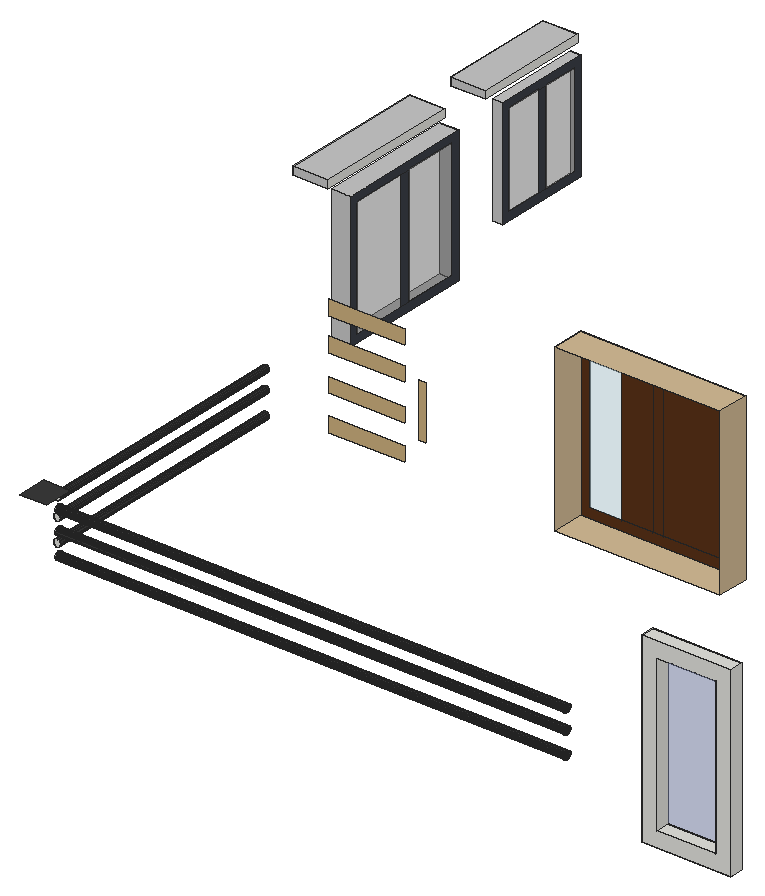
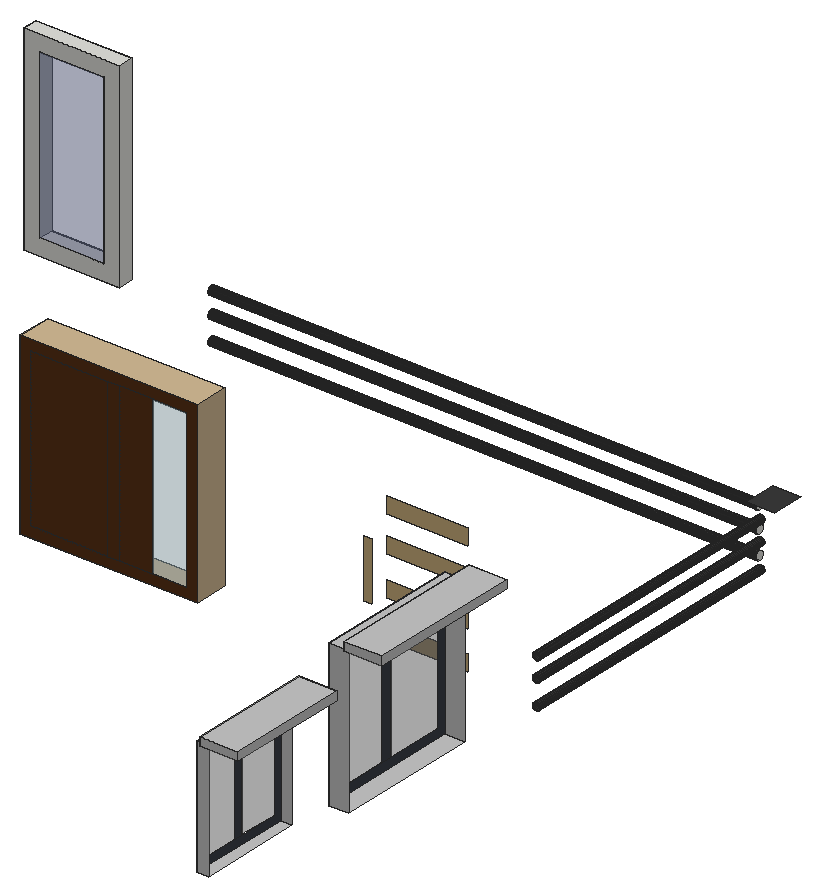
# SketchUp Ruby script. Lengths in inches.
U = 1.inch
M = Sketchup.active_model
def pt(a) = Geom::Point3d.new(a.map { |v| v * U })
def face(e, loops, mat)
  f = e.add_face(loops[0].map { |a| pt(a) })
  loops[1..].each { |l| e.add_face(l.map { |a| pt(a) }).erase! }
  f.material = f.back_material = mat if mat
  f
end
# faces: each face lists its corners as indices into pts; further lists are holes
def faces(e, pts, list, mat = nil) = list.each { |f| face(e, (f[0].is_a?(Array) ? f : [f]).map { |l| l.map { |i| pts[i] } }, mat) }
# xy, xz, yz: faces in a plane at the given z, y or x. An outline is a flat list of corners, or four numbers for a rectangle; further outlines are holes
def ring(l) = l.size == 4 ? [[l[0], l[1]], [l[2], l[1]], [l[2], l[3]], [l[0], l[3]]] : l.each_slice(2).to_a
def flat(e, list, mat, &to3) = list.each { |f| face(e, (f[0].is_a?(Array) ? f : [f]).map { |l| ring(l).map { |u, v| to3.(u, v) } }, mat) }
def xy(e, z, list, mat = nil) = flat(e, list, mat) { |x, y| [x, y, z] }
def xz(e, y, list, mat = nil) = flat(e, list, mat) { |x, z| [x, y, z] }
def yz(e, x, list, mat = nil) = flat(e, list, mat) { |y, z| [x, y, z] }
def lines(e, pts, list) = list.each { |a, b| e.add_line(pt(pts[a]), pt(pts[b])) }
# prism: a flat outline (further loops are holes) pulled along v
def prism(e, loops, v, mat = nil)
  f = face(e, loops, mat); d = Geom::Vector3d.new(v.map { |x| x * U })
  f.pushpull(f.normal.samedirection?(d) ? d.length : -d.length)
end
def box(e, o, s, mat = nil) = prism(e, [[o, [o[0] + s[0], o[1], o[2]], [o[0] + s[0], o[1] + s[1], o[2]], [o[0], o[1] + s[1], o[2]]]], [0, 0, s[2]], mat)
def at(x, y, z, deg = 0) = Geom::Transformation.translation(pt([x, y, z])) * Geom::Transformation.rotation(ORIGIN, Z_AXIS, deg.degrees)
def axes(o, x, y, z) = Geom::Transformation.new([*x, 0, *y, 0, *z, 0, *pt(o).to_a, 1])
def part(name) = M.definitions.add(name)
# library, detail: a bought-in or finely detailed component or shape, given as its bounding box
def library(name, o, s) = part(name).tap { |d| box(d.entities, o, s) }
def detail(e, o, s) = box(e.add_group.entities, o, s)
def put(e, d, t, mat = nil) = e.add_instance(d, t).tap { |i| i.material = mat if mat }
def group(e, t, mat = nil) = e.add_group.tap { |g| g.transformation = t; g.material = mat if mat }.entities
root = M.entities
M.materials.add("[Color M02]").color = [198, 198, 198]
M.materials.add("[Color M07]").color = [58, 58, 58]
M.materials.add("[Formica Beige]").color = [211, 187, 149]
M.materials.add("[Formica Laminate Dark]").color = [59, 63, 71]
M.materials.add("[Translucent Glass Gray]").color = [128, 128, 128]
M.materials["[Translucent Glass Gray]"].alpha = 0.5
M.materials.add("[Translucent Glass Safety]").color = [204, 235, 244]
M.materials["[Translucent Glass Safety]"].alpha = 0.5
M.materials.add("[Translucent Glass Sky Reflection]").color = [126, 138, 183]
M.materials["[Translucent Glass Sky Reflection]"].alpha = 0.52
M.materials.add("[Wood Cherry Original]").color = [89, 50, 24]
M.materials.add("[Wood Floor Light]").color = [204, 176, 127]
xy(root,406.1,[[374.52,386.84,415.58,393.34]])
xy(root,411.53,[[213.51,538.2,289.58,552.88]],"[Formica Beige]")
xy(root,412.93,[[381.35,386.84,408.75,393.34]])
xy(root,421.07,[[73.92,584.23,82.36,646.54]],"[Color M02]")
xy(root,429.73,[[73.92,676.68,78.67,721.56]],"[Color M02]")
xy(root,431,[[79.95,477.84,80.34,477.9,80.7,478.05,81.01,478.28,81.25,478.59,81.4,478.96,81.45,479.34,81.4,479.73,81.25,480.09,81.01,480.41,80.7,480.64,80.34,480.79,79.95,480.84,79.5625,480.79,79.2,480.64,78.89,480.41,78.65,480.09,78.5,479.73,78.45,479.34,78.5,478.96,78.65,478.59,78.89,478.28,79.2,478.05,79.5625,477.9]])
xy(root,431.16,[[79.95,444.41,80.34,444.46,80.7,444.61,81.01,444.85,81.25,445.16,81.4,445.52,81.45,445.91,81.4,446.3,81.25,446.66,81.01,446.97,80.7,447.21,80.34,447.36,79.95,447.41,79.5625,447.36,79.2,447.21,78.89,446.97,78.65,446.66,78.5,446.3,78.45,445.91,78.5,445.52,78.65,445.16,78.89,444.85,79.2,444.61,79.5625,444.46]])
xy(root,431.4375,[[193.34,408.87,193.78,408.93,194.18,409.1,194.53,409.36,194.8,409.71,194.97,410.12,195.03,410.56,194.97,410.99,194.8,411.4,194.53,411.75,194.18,412.02,193.78,412.1875,193.34,412.25,192.9,412.1875,192.5,412.02,192.15,411.75,191.88,411.4,191.71,410.99,191.65,410.56,191.71,410.12,191.88,409.71,192.15,409.36,192.5,409.1,192.9,408.93]])
xy(root,431.5625,[[259.47,408.87,259.9,408.93,260.31,409.1,260.66,409.36,260.93,409.71,261.1,410.12,261.15,410.56,261.1,410.99,260.93,411.4,260.66,411.75,260.31,412.02,259.9,412.1875,259.47,412.25,259.03,412.1875,258.62,412.02,258.27,411.75,258,411.4,257.84,410.99,257.78,410.56,257.84,410.12,258,409.71,258.27,409.36,258.62,409.1,259.03,408.93]])
xy(root,431.75,[[128.47,408.87,128.9,408.93,129.31,409.1,129.66,409.36,129.93,409.71,130.1,410.12,130.15,410.56,130.1,410.99,129.93,411.4,129.66,411.75,129.31,412.02,128.9,412.1875,128.47,412.25,128.03,412.1875,127.62,412.02,127.27,411.75,127,411.4,126.84,410.99,126.78,410.56,126.84,410.12,127,409.71,127.27,409.36,127.62,409.1,128.03,408.93]])
xy(root,431.875,[[79.95,511.66,80.34,511.71,80.7,511.86,81.01,512.1,81.25,512.41,81.4,512.77,81.45,513.16,81.4,513.55,81.25,513.91,81.01,514.22,80.7,514.46,80.34,514.61,79.95,514.66,79.5625,514.61,79.2,514.46,78.89,514.22,78.65,513.91,78.5,513.55,78.45,513.16,78.5,512.77,78.65,512.41,78.89,512.1,79.2,511.86,79.5625,511.71]])
xy(root,436.0625,[[73.92,404.34,85.98,418.04]],"[Color M07]")
xy(root,480.23,[[73.92,676.68,78.67,721.56]],"[Color M02]")
xy(root,481.56,[[57.67,672.99,73.92,725.89]],"[Color M02]")
xy(root,483.38,[[73.92,584.23,82.36,646.54]],"[Color M02]")
xy(root,484.43,[[57.67,581.95,73.92,649.2]],"[Color M02]")
xy(root,484.52,[[381.35,386.84,408.75,393.34]])
xy(root,485.25,[[57.67,672.99,73.92,725.89]],"[Color M02]")
xy(root,487.59,[[213.51,538.2,289.58,552.88]],"[Formica Beige]")
xy(root,488.12,[[57.67,581.95,73.92,649.2]],"[Color M02]")
xy(root,491.35,[[374.52,386.84,415.58,393.34]])
xz(root,386.84,[[[374.52,406.1,415.58,491.35],[381.35,412.93,408.75,484.52]]])
xz(root,393.34,[[[374.52,406.1,415.58,491.35],[381.35,412.93,408.75,484.52]]])
xz(root,393.34,[[381.35,412.93,408.75,484.52]],"[Translucent Glass Sky Reflection]")
xz(root,418.04,[[80,410.64,80.42,410.7,80.81,410.86,81.15,411.12,81.4,411.45,81.57,411.85,81.62,412.27,81.57,412.6875,81.4,413.08,81.15,413.42,80.81,413.67,80.42,413.84,80,413.89,79.58,413.84,79.18,413.67,78.85,413.42,78.59,413.08,78.43,412.6875,78.37,412.27,78.43,411.85,78.59,411.45,78.85,411.12,79.18,410.86,79.58,410.7],[80,421.33,80.42,421.39,80.81,421.55,81.15,421.81,81.4,422.14,81.57,422.53,81.62,422.95,81.57,423.375,81.4,423.77,81.15,424.1,80.81,424.36,80.42,424.52,80,424.58,79.58,424.52,79.18,424.36,78.85,424.1,78.59,423.77,78.43,423.375,78.37,422.95,78.43,422.53,78.59,422.14,78.85,421.81,79.18,421.55,79.58,421.39],[80,429.95,80.42,430.01,80.81,430.17,81.15,430.43,81.4,430.77,81.57,431.16,81.62,431.58,81.57,432,81.4,432.39,81.15,432.73,80.81,432.99,80.42,433.15,80,433.2,79.58,433.15,79.18,432.99,78.85,432.73,78.59,432.39,78.43,432,78.37,431.58,78.43,431.16,78.59,430.77,78.85,430.43,79.18,430.17,79.58,430.01]])
xz(root,538.2,[[109.29,415.48,144.04,422.29],[150.7,427.01,154.02,451.83],[109.29,431.66,144.04,438.48],[109.29,448.48,144.04,455.29],[109.29,463.85,144.04,470.66]],"[Wood Floor Light]")
xz(root,552.88,[[217.97,415.98,232.47,483.13]],"[Translucent Glass Safety]")
xz(root,552.88,[[[213.51,411.53,289.58,487.59],[217.97,415.98,285.12,483.13]],[232.47,415.98,246.96,483.13],[246.96,415.98,251.87,483.13],[251.87,415.98,285.12,483.13]],"[Wood Cherry Original]")
xz(root,581.95,[[57.67,484.43,73.92,488.12]],"[Color M02]")
xz(root,584.23,[[73.92,421.07,82.36,483.38]],"[Color M02]")
xz(root,646.54,[[73.92,421.07,82.36,483.38]],"[Color M02]")
xz(root,649.2,[[57.67,484.43,73.92,488.12]],"[Color M02]")
xz(root,672.99,[[57.67,481.56,73.92,485.25]],"[Color M02]")
xz(root,676.68,[[73.92,429.73,78.67,480.23]],"[Color M02]")
xz(root,721.56,[[73.92,429.73,78.67,480.23]],"[Color M02]")
xz(root,725.89,[[57.67,481.56,73.92,485.25]],"[Color M02]")
yz(root,57.67,[[672.99,481.56,725.89,485.25],[581.95,484.43,649.2,488.12]],"[Color M02]")
yz(root,73.92,[[672.99,481.56,725.89,485.25],[581.95,484.43,649.2,488.12]])
yz(root,78.67,[[[676.68,429.73,721.56,480.23],[680.29,433.34,717.95,476.63]],[697.6,433.34,701.4,476.63]],"[Formica Laminate Dark]")
yz(root,78.67,[[680.29,433.34,697.6,476.63],[701.4,433.34,717.95,476.63]],"[Translucent Glass Gray]")
yz(root,82.36,[[[584.23,421.07,646.54,483.38],[587.9,424.74,642.87,479.71]],[613.09,424.74,618.09,479.71]],"[Formica Laminate Dark]")
yz(root,82.36,[[587.9,424.74,613.09,479.71],[618.09,424.74,642.87,479.71]],"[Translucent Glass Gray]")
yz(root,85.98,[[411.11,410.55,410.66,410.61,410.24,410.79,409.875,411.07,409.6,411.43,409.42,411.85,409.36,412.3,409.42,412.76,409.6,413.18,409.875,413.54,410.24,413.82,410.66,414,411.11,414.05,411.57,414,411.99,413.82,412.35,413.54,412.63,413.18,412.8,412.76,412.86,412.3,412.8,411.85,412.63,411.43,412.35,411.07,411.99,410.79,411.57,410.61],[411.11,420.8,410.66,420.86,410.24,421.04,409.875,421.32,409.6,421.68,409.42,422.1,409.36,422.55,409.42,423.01,409.6,423.43,409.875,423.79,410.24,424.07,410.66,424.25,411.11,424.3,411.57,424.25,411.99,424.07,412.35,423.79,412.63,423.43,412.8,423.01,412.86,422.55,412.8,422.1,412.63,421.68,412.35,421.32,411.99,421.04,411.57,420.86],[411.11,429.99,410.66,430.05,410.24,430.23,409.875,430.51,409.6,430.87,409.42,431.29,409.36,431.74,409.42,432.2,409.6,432.62,409.875,432.98,410.24,433.26,410.66,433.43,411.11,433.49,411.57,433.43,411.99,433.26,412.35,432.98,412.63,432.62,412.8,432.2,412.86,431.74,412.8,431.29,412.63,430.87,412.35,430.51,411.99,430.23,411.57,430.05]])
yz(root,213.51,[[538.2,411.53,552.88,487.59]],"[Formica Beige]")
yz(root,289.58,[[538.2,411.53,552.88,487.59]],"[Formica Beige]")
yz(root,374.52,[[386.84,406.1,393.34,491.35]])
yz(root,381.35,[[386.84,412.93,393.34,484.52]])
yz(root,408.75,[[386.84,412.93,393.34,484.52]])
yz(root,415.58,[[386.84,406.1,393.34,491.35]])
p = [[85.98,410.24,410.79],[85.98,410.66,410.61],[320.99,410.66,410.61],[320.99,410.24,410.79],[85.98,411.11,410.55],[320.99,411.11,410.55],
  [85.98,411.57,410.61],[320.99,411.57,410.61],[85.98,411.99,410.79],[320.99,411.99,410.79],[80,418.04,410.64],[79.58,418.04,410.7],
  [79.58,538.2,410.7],[80,538.2,410.64],[80.42,418.04,410.7],[80.42,538.2,410.7],[79.18,418.04,410.86],[79.18,538.2,410.86],
  [80.81,418.04,410.86],[80.81,538.2,410.86],[85.98,409.875,411.07],[320.99,409.875,411.07],[85.98,412.35,411.07],[320.99,412.35,411.07],
  [78.85,418.04,411.12],[78.85,538.2,411.12],[81.15,418.04,411.12],[81.15,538.2,411.12],[85.98,409.6,411.43],[320.99,409.6,411.43],
  [85.98,412.63,411.43],[320.99,412.63,411.43],[78.59,418.04,411.45],[78.59,538.2,411.45],[81.4,418.04,411.45],[81.4,538.2,411.45],
  [85.98,409.42,411.85],[320.99,409.42,411.85],[85.98,412.8,411.85],[320.99,412.8,411.85],[78.43,418.04,411.85],[78.43,538.2,411.85],
  [81.57,418.04,411.85],[81.57,538.2,411.85],[78.37,418.04,412.27],[78.37,538.2,412.27],[81.62,418.04,412.27],[81.62,538.2,412.27],
  [85.98,409.36,412.3],[320.99,409.36,412.3],[85.98,412.86,412.3],[320.99,412.86,412.3],[85.98,409.42,412.76],[320.99,409.42,412.76],
  [85.98,412.8,412.76],[320.99,412.8,412.76],[78.43,418.04,412.6875],[78.43,538.2,412.6875],[81.57,418.04,412.6875],[81.57,538.2,412.6875],
  [78.59,418.04,413.08],[78.59,538.2,413.08],[81.4,418.04,413.08],[81.4,538.2,413.08],[85.98,409.6,413.18],[320.99,409.6,413.18],
  [85.98,412.63,413.18],[320.99,412.63,413.18],[78.85,418.04,413.42],[78.85,538.2,413.42],[81.15,418.04,413.42],[81.15,538.2,413.42],
  [85.98,409.875,413.54],[320.99,409.875,413.54],[85.98,412.35,413.54],[320.99,412.35,413.54],[79.18,418.04,413.67],[79.18,538.2,413.67],
  [80.81,418.04,413.67],[80.81,538.2,413.67],[85.98,410.24,413.82],[320.99,410.24,413.82],[85.98,411.99,413.82],[320.99,411.99,413.82],
  [79.58,418.04,413.84],[79.58,538.2,413.84],[80.42,418.04,413.84],[80.42,538.2,413.84],[85.98,410.66,414],[320.99,410.66,414],
  [85.98,411.57,414],[320.99,411.57,414],[80,418.04,413.89],[80,538.2,413.89],[85.98,411.11,414.05],[320.99,411.11,414.05],
  [85.98,410.66,420.86],[85.98,411.11,420.8],[320.99,411.11,420.8],[320.99,410.66,420.86],[85.98,411.57,420.86],[320.99,411.57,420.86],
  [85.98,410.24,421.04],[320.99,410.24,421.04],[85.98,411.99,421.04],[320.99,411.99,421.04],[85.98,409.875,421.32],[320.99,409.875,421.32],
  [85.98,412.35,421.32],[320.99,412.35,421.32],[85.98,409.6,421.68],[320.99,409.6,421.68],[85.98,412.63,421.68],[320.99,412.63,421.68],
  [80,418.04,421.33],[79.58,418.04,421.39],[79.58,538.2,421.39],[80,538.2,421.33],[80.42,418.04,421.39],[80.42,538.2,421.39],
  [79.18,418.04,421.55],[79.18,538.2,421.55],[80.81,418.04,421.55],[80.81,538.2,421.55],[78.85,418.04,421.81],[78.85,538.2,421.81],
  [81.15,418.04,421.81],[81.15,538.2,421.81],[85.98,409.42,422.1],[320.99,409.42,422.1],[85.98,412.8,422.1],[320.99,412.8,422.1],
  [78.59,418.04,422.14],[78.59,538.2,422.14],[81.4,418.04,422.14],[81.4,538.2,422.14],[85.98,409.36,422.55],[320.99,409.36,422.55],
  [85.98,412.86,422.55],[320.99,412.86,422.55],[78.43,418.04,422.53],[78.43,538.2,422.53],[81.57,418.04,422.53],[81.57,538.2,422.53],
  [78.37,418.04,422.95],[78.37,538.2,422.95],[81.62,418.04,422.95],[81.62,538.2,422.95],[85.98,409.42,423.01],[320.99,409.42,423.01],
  [85.98,412.8,423.01],[320.99,412.8,423.01],[85.98,409.6,423.43],[320.99,409.6,423.43],[85.98,412.63,423.43],[320.99,412.63,423.43],
  [78.43,418.04,423.375],[78.43,538.2,423.375],[81.57,418.04,423.375],[81.57,538.2,423.375],[85.98,409.875,423.79],[320.99,409.875,423.79],
  [85.98,412.35,423.79],[320.99,412.35,423.79],[78.59,418.04,423.77],[78.59,538.2,423.77],[81.4,418.04,423.77],[81.4,538.2,423.77],
  [85.98,410.24,424.07],[320.99,410.24,424.07],[85.98,411.99,424.07],[320.99,411.99,424.07],[78.85,418.04,424.1],[78.85,538.2,424.1],
  [81.15,418.04,424.1],[81.15,538.2,424.1],[85.98,410.66,424.25],[320.99,410.66,424.25],[85.98,411.57,424.25],[320.99,411.57,424.25],
  [79.18,418.04,424.36],[79.18,538.2,424.36],[80.81,418.04,424.36],[80.81,538.2,424.36],[85.98,411.11,424.3],[320.99,411.11,424.3],
  [79.58,418.04,424.52],[79.58,538.2,424.52],[80.42,418.04,424.52],[80.42,538.2,424.52],[80,418.04,424.58],[80,538.2,424.58],
  [85.98,410.66,430.05],[85.98,411.11,429.99],[320.99,411.11,429.99],[320.99,410.66,430.05],[85.98,411.57,430.05],[320.99,411.57,430.05],
  [79.58,418.04,430.01],[79.18,418.04,430.17],[79.18,538.2,430.17],[79.58,538.2,430.01],[80,418.04,429.95],[80,538.2,429.95],
  [80.42,418.04,430.01],[80.42,538.2,430.01],[80.81,418.04,430.17],[80.81,538.2,430.17],[85.98,410.24,430.23],[320.99,410.24,430.23],
  [85.98,411.99,430.23],[320.99,411.99,430.23],[85.98,409.875,430.51],[320.99,409.875,430.51],[85.98,412.35,430.51],[320.99,412.35,430.51],
  [78.85,418.04,430.43],[78.85,538.2,430.43],[81.15,418.04,430.43],[81.15,538.2,430.43],[78.59,418.04,430.77],[78.59,538.2,430.77],
  [81.4,418.04,430.77],[81.4,538.2,430.77],[85.98,409.6,430.87],[320.99,409.6,430.87],[85.98,412.63,430.87],[320.99,412.63,430.87],
  [78.43,418.04,431.16],[78.43,538.2,431.16],[81.57,418.04,431.16],[81.57,538.2,431.16],[85.98,409.42,431.29],[320.99,409.42,431.29],
  [85.98,412.8,431.29],[320.99,412.8,431.29],[78.37,418.04,431.58],[78.37,538.2,431.58],[81.62,418.04,431.58],[81.62,538.2,431.58],
  [85.98,409.36,431.74],[320.99,409.36,431.74],[85.98,412.86,431.74],[320.99,412.86,431.74],[78.43,418.04,432],[78.43,538.2,432],
  [81.57,418.04,432],[81.57,538.2,432],[85.98,409.42,432.2],[320.99,409.42,432.2],[85.98,412.8,432.2],[320.99,412.8,432.2],
  [78.59,418.04,432.39],[78.59,538.2,432.39],[81.4,418.04,432.39],[81.4,538.2,432.39],[85.98,409.6,432.62],[320.99,409.6,432.62],
  [85.98,412.63,432.62],[320.99,412.63,432.62],[78.85,418.04,432.73],[78.85,538.2,432.73],[81.15,418.04,432.73],[81.15,538.2,432.73],
  [85.98,409.875,432.98],[320.99,409.875,432.98],[85.98,412.35,432.98],[320.99,412.35,432.98],[79.18,418.04,432.99],[79.18,538.2,432.99],
  [80.81,418.04,432.99],[80.81,538.2,432.99],[85.98,410.24,433.26],[320.99,410.24,433.26],[85.98,411.99,433.26],[320.99,411.99,433.26],
  [79.58,418.04,433.15],[79.58,538.2,433.15],[80.42,418.04,433.15],[80.42,538.2,433.15],[80,418.04,433.2],[80,538.2,433.2],
  [85.98,410.66,433.43],[320.99,410.66,433.43],[85.98,411.57,433.43],[320.99,411.57,433.43],[85.98,411.11,433.49],[320.99,411.11,433.49]]
faces(root,p,[[0,1,2,3],[1,4,5,2],[4,6,7,5],[6,8,9,7],[10,11,12,13],[14,10,13,15],[11,16,17,12],[18,14,15,19],
  [20,0,3,21],[8,22,23,9],[16,24,25,17],[26,18,19,27],[28,20,21,29],[22,30,31,23],[24,32,33,25],[34,26,27,35],
  [36,28,29,37],[30,38,39,31],[32,40,41,33],[42,34,35,43],[40,44,45,41],[46,42,43,47],[48,36,37,49],[38,50,51,39],
  [52,48,49,53],[50,54,55,51],[44,56,57,45],[58,46,47,59],[56,60,61,57],[62,58,59,63],[64,52,53,65],[54,66,67,55],
  [60,68,69,61],[70,62,63,71],[72,64,65,73],[66,74,75,67],[68,76,77,69],[78,70,71,79],[80,72,73,81],[74,82,83,75],
  [76,84,85,77],[86,78,79,87],[88,80,81,89],[82,90,91,83],[84,92,93,85],[92,86,87,93],[94,88,89,95],[90,94,95,91],
  [96,97,98,99],[97,100,101,98],[102,96,99,103],[100,104,105,101],[106,102,103,107],[104,108,109,105],[110,106,107,111],[108,112,113,109],
  [114,115,116,117],[118,114,117,119],[115,120,121,116],[122,118,119,123],[120,124,125,121],[126,122,123,127],[128,110,111,129],[112,130,131,113],
  [124,132,133,125],[134,126,127,135],[136,128,129,137],[130,138,139,131],[132,140,141,133],[142,134,135,143],[140,144,145,141],[146,142,143,147],
  [148,136,137,149],[138,150,151,139],[152,148,149,153],[150,154,155,151],[144,156,157,145],[158,146,147,159],[160,152,153,161],[154,162,163,155],
  [156,164,165,157],[166,158,159,167],[168,160,161,169],[162,170,171,163],[164,172,173,165],[174,166,167,175],[176,168,169,177],[170,178,179,171],
  [172,180,181,173],[182,174,175,183],[184,176,177,185],[178,184,185,179],[180,186,187,181],[188,182,183,189],[186,190,191,187],[190,188,189,191],
  [192,193,194,195],[193,196,197,194],[198,199,200,201],[202,198,201,203],[204,202,203,205],[206,204,205,207],[208,192,195,209],[196,210,211,197],
  [212,208,209,213],[210,214,215,211],[199,216,217,200],[218,206,207,219],[216,220,221,217],[222,218,219,223],[224,212,213,225],[214,226,227,215],
  [220,228,229,221],[230,222,223,231],[232,224,225,233],[226,234,235,227],[228,236,237,229],[238,230,231,239],[240,232,233,241],[234,242,243,235],
  [236,244,245,237],[246,238,239,247],[248,240,241,249],[242,250,251,243],[244,252,253,245],[254,246,247,255],[256,248,249,257],[250,258,259,251],
  [252,260,261,253],[262,254,255,263],[264,256,257,265],[258,266,267,259],[260,268,269,261],[270,262,263,271],[272,264,265,273],[266,274,275,267],
  [268,276,277,269],[278,270,271,279],[276,280,281,277],[280,278,279,281],[282,272,273,283],[274,284,285,275],[286,282,283,287],[284,286,287,285]],"[Color M07]")
